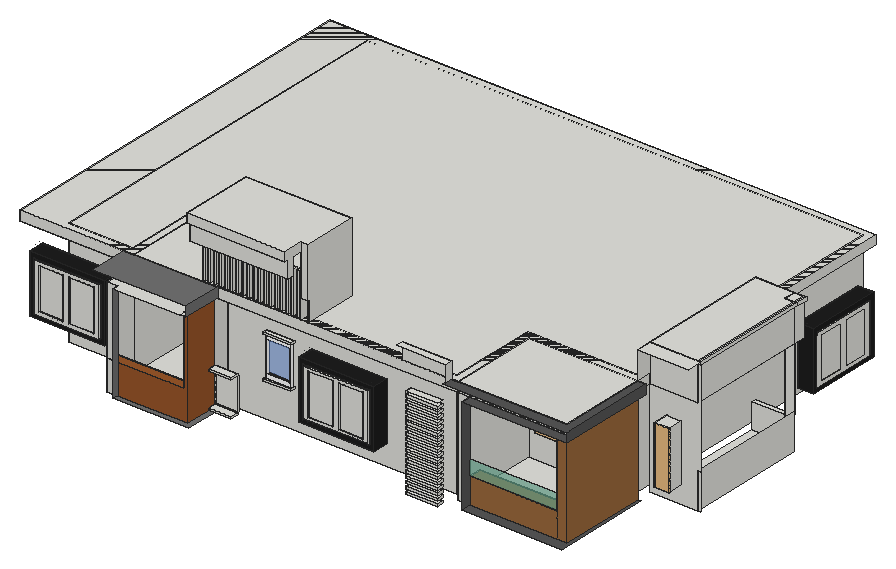
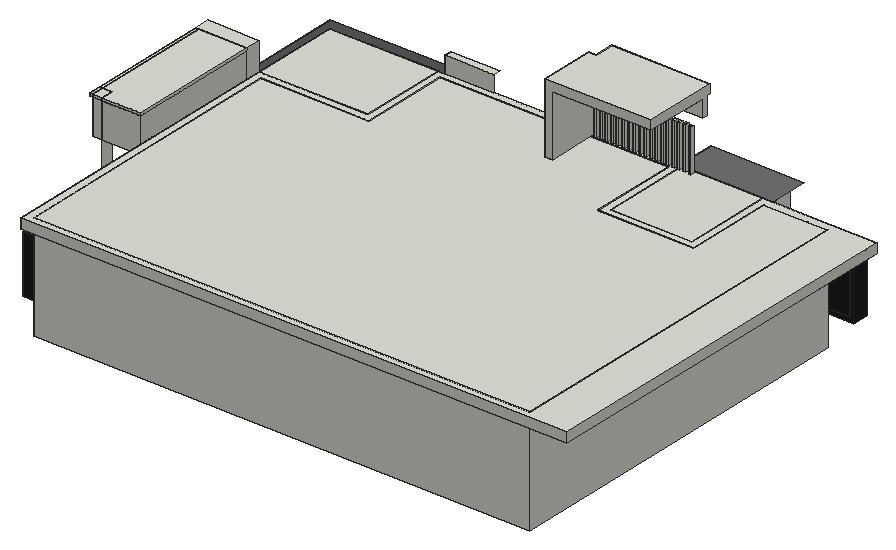
# SketchUp Ruby script. Lengths in inches.
U = 1.inch
M = Sketchup.active_model
def pt(a) = Geom::Point3d.new(a.map { |v| v * U })
def face(e, loops, mat)
  f = e.add_face(loops[0].map { |a| pt(a) })
  loops[1..].each { |l| e.add_face(l.map { |a| pt(a) }).erase! }
  f.material = f.back_material = mat if mat
  f
end
# faces: each face lists its corners as indices into pts; further lists are holes
def faces(e, pts, list, mat = nil) = list.each { |f| face(e, (f[0].is_a?(Array) ? f : [f]).map { |l| l.map { |i| pts[i] } }, mat) }
# xy, xz, yz: faces in a plane at the given z, y or x. An outline is a flat list of corners, or four numbers for a rectangle; further outlines are holes
def ring(l) = l.size == 4 ? [[l[0], l[1]], [l[2], l[1]], [l[2], l[3]], [l[0], l[3]]] : l.each_slice(2).to_a
def flat(e, list, mat, &to3) = list.each { |f| face(e, (f[0].is_a?(Array) ? f : [f]).map { |l| ring(l).map { |u, v| to3.(u, v) } }, mat) }
def xy(e, z, list, mat = nil) = flat(e, list, mat) { |x, y| [x, y, z] }
def xz(e, y, list, mat = nil) = flat(e, list, mat) { |x, z| [x, y, z] }
def yz(e, x, list, mat = nil) = flat(e, list, mat) { |y, z| [x, y, z] }
def lines(e, pts, list) = list.each { |a, b| e.add_line(pt(pts[a]), pt(pts[b])) }
# prism: a flat outline (further loops are holes) pulled along v
def prism(e, loops, v, mat = nil)
  f = face(e, loops, mat); d = Geom::Vector3d.new(v.map { |x| x * U })
  f.pushpull(f.normal.samedirection?(d) ? d.length : -d.length)
end
def box(e, o, s, mat = nil) = prism(e, [[o, [o[0] + s[0], o[1], o[2]], [o[0] + s[0], o[1] + s[1], o[2]], [o[0], o[1] + s[1], o[2]]]], [0, 0, s[2]], mat)
def at(x, y, z, deg = 0) = Geom::Transformation.translation(pt([x, y, z])) * Geom::Transformation.rotation(ORIGIN, Z_AXIS, deg.degrees)
def axes(o, x, y, z) = Geom::Transformation.new([*x, 0, *y, 0, *z, 0, *pt(o).to_a, 1])
def part(name) = M.definitions.add(name)
# library, detail: a bought-in or finely detailed component or shape, given as its bounding box
def library(name, o, s) = part(name).tap { |d| box(d.entities, o, s) }
def detail(e, o, s) = box(e.add_group.entities, o, s)
def put(e, d, t, mat = nil) = e.add_instance(d, t).tap { |i| i.material = mat if mat }
def group(e, t, mat = nil) = e.add_group.tap { |g| g.transformation = t; g.material = mat if mat }.entities
root = M.entities
M.materials.add("MaterialE").color = [182, 131, 172]
M.materials["MaterialE"].alpha = 0.66
M.materials.add("MaterialF").color = [114, 188, 161]
M.materials["MaterialF"].alpha = 0.66
M.materials.add("[Color M05]").color = [114, 114, 114]
M.materials.add("[Color M06]").color = [86, 86, 86]
M.materials.add("[Color M08]").color = [30, 30, 30]
M.materials.add("[Color_000]").color = [255, 255, 255]
M.materials.add("[Translucent Glass Blue]").color = [100, 149, 237]
M.materials["[Translucent Glass Blue]"].alpha = 0.5
M.materials.add("[Wood Cherry Original]").color = [152, 86, 42]
M.materials.add("[Wood Floor]").color = [155, 105, 61]
c1 = part("Group\#4")
box(c1.entities,[0,0,0],[39.5625,8.625,2.78])
c2 = part("Group\#75")
box(c2.entities,[0,-10.375,0],[28.375,10.375,2.5])
c3 = library("Single door",[0,0,0],[7.5,39.86,83.92])
c4 = part("Window")
xy(c4.entities,31.72,[[-0.78,88.6,2.72,128.1]])
xy(c4.entities,34.95,[[-0.78,91.53,0.84,106.59],[0.84,91.53,1.05,97.58],[1.05,91.53,1.42,106.59],[1.42,91.53,2.72,106.59],[0.84,97.58,1.05,98.18],
  [0.84,98.18,1.05,106.59]])
xy(c4.entities,35.27,[[-0.78,110.09,0.97,125.14],[1.05,110.09,2.72,125.14]])
xy(c4.entities,58.35,[[2.72,108.74,3.8,109.74]])
xy(c4.entities,77.8125,[[-0.78,110.09,2.72,125.14],[0.97,110.09,1.05,125.14]])
xy(c4.entities,77.93,[[-0.78,91.53,0.84,106.59],[1.05,91.53,1.42,106.59],[1.42,91.53,2.72,106.59]])
xy(c4.entities,80.72,[[-0.78,88.6,2.72,128.1]])
xz(c4.entities,88.6,[[-0.78,31.72,2.72,80.72]])
xz(c4.entities,91.53,[[-0.78,34.95,0.84,77.93],[1.05,34.95,1.42,77.93],[1.42,34.95,2.72,77.93]])
xz(c4.entities,106.59,[[-0.78,34.95,0.84,77.93],[0.84,34.95,1.05,77.93],[0.84,34.95,2.72,77.93]])
xz(c4.entities,108.74,[[3.8,54.35,4.22,54.6,4.22,59.47,2.72,59.97,2.72,58.35,3.8,58.35]])
xz(c4.entities,109.74,[[3.8,54.35,3.8,58.35,2.72,58.35,2.72,59.97,4.22,59.47,4.22,54.6]])
xz(c4.entities,110.09,[[-0.78,35.27,0.97,77.8125],[1.05,35.27,2.72,77.8125]])
xz(c4.entities,125.14,[[-0.78,35.27,0.97,77.8125],[0.97,35.27,1.05,80.72],[1.05,35.27,2.72,77.8125]])
xz(c4.entities,128.1,[[-0.78,31.72,2.72,80.72]])
yz(c4.entities,-0.78,[[[88.6,31.72,128.1,80.72],[91.53,34.95,106.59,77.93],[110.09,35.27,125.14,77.8125]]])
yz(c4.entities,0.84,[[91.53,34.95,106.59,77.93]])
yz(c4.entities,0.97,[[110.09,35.27,125.14,77.8125]])
yz(c4.entities,1.05,[[91.53,34.95,106.59,77.93],[110.09,35.27,125.14,77.8125]])
yz(c4.entities,1.42,[[91.53,34.95,106.59,77.93]])
yz(c4.entities,2.72,[[[88.6,31.72,108.35,80.72],[91.53,34.95,106.59,77.93]],[[108.35,31.72,128.1,80.72],[110.09,35.27,125.14,77.8125],[108.74,58.35,109.74,59.97]]])
yz(c4.entities,3.8,[[108.74,54.35,109.74,58.35]])
yz(c4.entities,4.22,[[108.74,54.6,109.74,59.47]])
p = [[4.22,108.74,54.6],[3.8,108.74,54.35],[3.8,109.74,54.35],[4.22,109.74,54.6],[2.72,109.74,59.97],[2.72,108.74,59.97],
  [4.22,108.74,59.47],[4.22,109.74,59.47],[-0.78,86.4,89.94],[-0.78,86.44,89.94],[15.22,130.69,89.94],[15.22,130.65,89.94],
  [-0.78,86.44,28.19],[-0.78,86.4,28.19],[7.72,130.69,89.94],[7.72,130.65,89.94]]
faces(c4.entities,p,[[0,1,2,3],[4,5,6,7]])
lines(c4.entities,p,[[8,9],[10,11],[12,13],[14,15]])
c5 = part("Group\#5")
xy(c5.entities,0,[[[0,0,93.5,72.0625],[5.4,5.4,88.1,66.66]],[5.4,5.4,88.1,66.66]])
xy(c5.entities,20.1875,[[[0,0,93.5,72.0625],[5.4,5.4,88.1,66.66]]])
xz(c5.entities,0,[[0,0,93.5,20.1875]])
xz(c5.entities,5.4,[[5.4,0,88.1,20.1875]])
xz(c5.entities,66.66,[[5.4,0,88.1,20.1875]])
xz(c5.entities,72.0625,[[0,0,93.5,20.1875]])
yz(c5.entities,0,[[0,0,72.0625,20.1875]])
yz(c5.entities,5.4,[[5.4,0,66.66,20.1875]])
yz(c5.entities,88.1,[[5.4,0,66.66,20.1875]])
yz(c5.entities,93.5,[[0,0,72.0625,20.1875]])
c6 = library("grille P1",[0,0,0],[0.79,28.9,72.83])
c7 = part("glassE")
xy(c7.entities,0,[[0,0,37.99,0.79]],"MaterialE")
xy(c7.entities,38.27,[[0,0,37.99,0.79]],"MaterialE")
xz(c7.entities,0,[[0,0,37.99,38.27]],"MaterialF")
yz(c7.entities,0,[[0,0,0.79,38.27]],"MaterialE")
yz(c7.entities,37.99,[[0,0,0.79,38.27]],"MaterialE")
c8 = library("Sliding Window",[0,0,0],[35.43,4.93,59.06])
c9 = part("Group\#73")
box(c9.entities,[0,0,0],[34.1875,2.25,6.125])
c10 = part("bod vindu")
g1 = group(c10.entities,at(0,-46.85,0),"[Translucent Glass Blue]")
yz(g1,0.94,[[2.36,2.36,44.49,19.65]],"[Translucent Glass Blue]")
p = [[0.55,44.49,2.36],[0.94,44.49,2.36],[0.55,2.36,19.65],[0.94,2.36,19.65]]
lines(g1,p,[[0,1],[2,3]])
g2 = group(g1,at(0,46.85,0,-90),"[Color_000]")
xy(g2,0,[[0,0,46.85,3.9375]])
xy(g2,1.57,[[1.57,0,45.28,0.55]])
xy(g2,2.36,[[2.36,0.55,44.49,3.9375]])
xy(g2,19.65,[[2.36,0.55,4.29,3.9375],[4.29,0.55,44.49,3.9375]])
xy(g2,20.43,[[1.57,0,45.28,0.55]])
xy(g2,22.01,[[0,0,46.85,3.9375]])
xz(g2,0,[[[0,0,46.85,22.01],[1.57,1.57,45.28,20.43]]])
xz(g2,0.55,[[1.57,1.57,45.28,2.36],[1.57,2.36,2.36,2.36,2.36,19.65,44.49,19.65,44.49,2.36,45.28,2.36,45.28,20.43,1.57,20.43]])
xz(g2,3.9375,[[[0,0,46.85,22.01],[2.36,2.36,44.49,19.65]]])
yz(g2,0,[[0,0,3.9375,22.01]])
yz(g2,1.57,[[0,1.57,0.55,2.36,0.55,20.43,0,20.43]])
yz(g2,2.36,[[0.55,2.36,3.9375,19.65]])
yz(g2,44.49,[[0.55,2.36,3.9375,19.65]])
yz(g2,45.28,[[0,1.57,0,20.43,0.55,20.43,0.55,2.36]])
yz(g2,46.85,[[0,0,3.9375,22.01]])
p = [[45.28,0,1.57],[1.57,0,1.57],[1.57,0.55,2.36],[2.36,0.55,2.36],[44.49,0.55,2.36],[45.28,0.55,2.36]]
faces(g2,p,[[0,1,2,3,4,5]])
xy(root,394.01,[[304.51,155.5,398.77,155.5,398.77,203.9375,392.02,203.9375,392.02,162.1875,291.51,162.1875,291.51,162.06,304.51,162.06]],"[Color M05]")
xy(root,396,[[291.51,172.6875,386.62,172.6875,386.62,203.9375,392.02,203.9375,392.02,313.75,291.32,313.75,291.32,203.9375,291.51,203.9375],[693.39,203.9375,707.82,203.9375,707.82,219.8125,816.38,219.8125,816.38,313.75,693.39,313.75],[203.47,212.9375,282.32,212.9375,282.32,322.75,401.02,322.75,401.02,212.9375,684.39,212.9375,684.39,322.75,818.97,322.75,818.97,674.9375,203.47,674.9375],[827.97,332.62,882.11,332.62,882.11,481.58,876.25,481.58,876.25,490.94,827.97,490.94],[882.11,332.62,887.97,481.58]])
xy(root,396,[[707.95,190.6875,832.47,190.6875,832.47,313.75,827.97,313.75,827.97,203.9375,707.95,203.9375]],"[Color M06]")
xy(root,397.79,[[392.02,203.9375,420.4,205.4375]])
xy(root,417.54,[[848.78,313.75,867.09,332.62]])
xy(root,426.875,[[827.97,490.94,876.25,496.51]])
xy(root,428,[[707.82,203.9375,816.38,219.8125]],"[Wood Floor]")
xy(root,432,[[291.51,162.1875,386.62,172.6875]],"[Wood Cherry Original]")
xy(root,438.17,[[392.02,203.9375,420.4,205.4375]])
xy(root,488.67,[[848.78,313.75,867.09,332.62]])
xy(root,501.53,[[635.73,194.4375,675.23,203.0625]])
xy(root,516,[[304.51,155.5,304.51,162.06,291.51,162.06,291.51,203.9375,386.62,203.9375,386.62,155.5],[386.62,155.5,392.02,162.1875],[386.62,162.1875,392.02,183],[386.62,183,392.02,203.9375],[816.38,203.9375,827.97,313.75],
  [827.97,332.62,887.97,496.51]])
xy(root,516,[[392.02,155.5,395.02,203.9375]],"[Color M05]")
xy(root,516,[[707.95,190.6875,707.95,203.9375,827.97,203.9375,827.97,313.75,838.2,313.75,838.2,190.6875]],"[Color M06]")
xy(root,528,[[[150.47,203.9375,291.32,203.9375,291.32,313.75,392.02,313.75,392.02,203.9375,693.39,203.9375,693.39,313.75,827.97,313.75,827.97,683.9375,150.47,683.9375],[203.47,212.9375,203.47,674.9375,818.97,674.9375,818.97,322.75,684.39,322.75,684.39,212.9375,401.02,212.9375,401.02,322.75,282.32,322.75,282.32,212.9375]],[497.83,203.9375,507.4,212.9375],[497.83,212.9375,507.4,271.6875]])
xy(root,528,[[278.57,155.5,395.02,203.9375]],"[Color M05]")
xy(root,528,[[685.61,190.6875,838.2,190.6875,838.2,313.75,827.97,313.75,827.97,203.9375,685.61,203.9375]],"[Color M06]")
xy(root,548.1875,[[624.38,194.4375,685.61,203.9375]])
xy(root,559.3125,[[827.97,332.62,827.97,496.51,876.25,496.51,876.25,481.58,887.97,481.58,887.97,332.62],[887.97,332.62,891.78,481.58],[876.25,481.58,887.97,496.51],[887.97,481.58,891.78,496.51]])
xy(root,562.75,[[827.97,313.75,891.78,332.62],[827.97,332.62,887.97,332.62,887.97,481.58,876.25,481.58,876.25,496.51,827.97,496.51],[887.97,332.62,891.78,481.58],[876.25,481.58,887.97,496.51],[887.97,481.58,891.78,496.51]])
xy(root,581.5,[[375.96,184.61,497.83,191.78]])
xy(root,603.3125,[[375.96,179.625,497.83,184.61],[375.96,191.78,497.83,203.9375],[375.96,203.9375,497.83,271.6875]])
xy(root,614.4375,[[375.96,179.625,497.83,179.625,497.83,203.9375,507.4,203.9375,507.4,271.6875,375.96,271.6875]])
xz(root,162.06,[[291.51,394.01,304.51,432],[291.51,432,304.51,516]])
xz(root,162.1875,[[291.51,394.01,392.02,394.01,392.02,516,386.62,516,386.62,432,291.51,432]],"[Wood Cherry Original]")
xz(root,172.6875,[[291.51,396,386.62,432]])
xz(root,179.625,[[375.96,603.3125,497.83,614.4375]])
xz(root,184.61,[[375.96,581.5,497.83,603.3125]])
xz(root,191.78,[[375.96,581.5,497.83,603.3125]])
xz(root,203.9375,[[291.32,396,291.32,528,392.02,528,392.02,516,291.51,516,291.51,396],[386.62,396,392.02,516],[693.39,396,693.39,528,827.97,528,827.97,516,707.95,516,707.95,428,707.82,428,707.82,396],[392.02,516,395.02,528],[507.4,528,508.2,552.375],
  [624.38,528,685.61,548.1875],[497.83,552.375,507.4,614.4375]])
xz(root,203.9375,[[707.95,396,816.38,428],[816.38,396,827.97,516]],"[Wood Floor]")
xz(root,205.4375,[[392.02,397.79,420.4,438.17]])
xz(root,212.9375,[[203.47,396,282.32,528],[401.02,396,684.39,528]])
xz(root,219.8125,[[707.82,396,816.38,428]])
xz(root,271.6875,[[497.83,528,497.83,603.3125,375.96,603.3125,375.96,614.4375,507.4,614.4375,507.4,528]])
xz(root,313.75,[[291.32,396,392.02,528],[693.39,396,816.38,528],[816.38,516,827.97,528]])
xz(root,313.75,[[827.97,516,838.2,528]],"[Color M06]")
xz(root,322.75,[[282.32,396,401.02,528],[684.39,396,818.97,528]])
xz(root,332.62,[[[827.97,396,827.97,516,887.97,516,887.97,559.3125,891.78,559.3125,891.78,441.07,887.97,441.07,887.97,396],[848.78,417.54,867.09,488.67]],[887.97,396,891.78,441.07],[827.97,516,887.97,559.3125],[827.97,559.3125,887.97,562.75],[887.97,559.3125,891.78,562.75]])
xz(root,481.58,[[876.25,396,887.97,559.3125],[876.25,559.3125,887.97,562.75],[887.97,559.3125,891.78,562.75]])
xz(root,490.94,[[827.97,396,876.25,426.875]])
xz(root,496.51,[[827.97,516,876.25,559.3125],[876.25,516,887.97,559.3125],[827.97,559.3125,876.25,562.75],[876.25,559.3125,887.97,562.75],[887.97,559.3125,891.78,562.75]])
xz(root,674.9375,[[203.47,396,818.97,528]])
yz(root,203.47,[[212.9375,396,674.9375,528]])
yz(root,282.32,[[212.9375,396,322.75,528]])
yz(root,291.32,[[203.9375,396,313.75,528]])
yz(root,291.51,[[162.06,394.01,162.1875,432],[172.6875,396,203.9375,396,203.9375,516,162.06,516,162.06,432,172.6875,432]])
yz(root,304.51,[[155.5,394.01,162.06,516]],"[Color M05]")
yz(root,375.96,[[184.61,581.5,184.61,603.3125,179.625,603.3125,179.625,614.4375,271.6875,614.4375,271.6875,603.3125,191.78,603.3125,191.78,581.5]])
yz(root,386.62,[[172.6875,396,172.6875,432,162.1875,432,162.1875,516,203.9375,516,203.9375,396]])
yz(root,392.02,[[203.9375,396,203.9375,397.79,205.4375,397.79,205.4375,438.17,203.9375,438.17,203.9375,528,313.75,528,313.75,396],[203.9375,397.79,205.4375,438.17],[203.9375,397.79,205.4375,438.17]])
yz(root,392.02,[[162.1875,394.01,203.9375,516]],"[Wood Cherry Original]")
yz(root,395.02,[[155.5,516,203.9375,528]],"[Color M05]")
yz(root,401.02,[[212.9375,396,322.75,528]])
yz(root,420.4,[[203.9375,397.79,205.4375,438.17]])
yz(root,497.83,[[203.9375,528,271.6875,603.3125],[184.61,581.5,191.78,581.5,191.78,603.3125,203.9375,603.3125,203.9375,614.4375,179.625,614.4375,179.625,603.3125,184.61,603.3125]])
yz(root,507.4,[[203.9375,528,271.6875,614.4375]])
yz(root,635.73,[[194.4375,497.67,203.0625,501.53]])
yz(root,684.39,[[212.9375,396,322.75,528]])
yz(root,685.61,[[194.4375,528,203.9375,548.1875]])
yz(root,693.39,[[203.9375,396,313.75,528]])
yz(root,707.82,[[203.9375,396,219.8125,428]])
yz(root,707.95,[[190.6875,396,203.9375,516]],"[Color M06]")
yz(root,816.38,[[219.8125,396,219.8125,428,203.9375,428,203.9375,516,313.75,516,313.75,396]],"[Wood Floor]")
yz(root,818.97,[[322.75,396,674.9375,528]])
yz(root,827.97,[[203.9375,516,313.75,528],[332.62,516,496.51,528],[313.75,528,332.62,562.75],[332.62,528,496.51,559.3125],[332.62,559.3125,496.51,562.75]])
yz(root,827.97,[[203.9375,396,313.75,516]],"[Wood Floor]")
yz(root,838.2,[[190.6875,516,313.75,528]],"[Color M06]")
yz(root,848.78,[[313.75,417.54,332.62,488.67]])
yz(root,867.09,[[313.75,417.54,332.62,488.67]])
yz(root,876.25,[[481.58,396,481.58,559.3125,496.51,559.3125,496.51,426.875,490.94,426.875,490.94,396],[481.58,559.3125,496.51,562.75]])
yz(root,887.97,[[332.62,396,481.58,441.07],[332.62,516,481.58,559.3125],[481.58,516,496.51,559.3125],[332.62,559.3125,481.58,562.75],[481.58,559.3125,496.51,562.75]])
yz(root,891.78,[[332.62,559.3125,481.58,562.75],[481.58,559.3125,496.51,562.75]])
p = [[291.32,203.9375,516],[291.51,183,516]]
lines(root,p,[[0,1]])
put(root,c1,at(635.73,194.4375,386.88))
put(root,c1,at(635.73,194.4375,392.88))
put(root,c2,at(392.02,203.9375,395.29))
put(root,c1,at(635.73,194.4375,398.88))
put(root,c3,at(760.44,316.08,402,-90))
put(root,c1,at(635.73,194.4375,404.88))
put(root,c1,at(635.73,194.4375,410.88))
put(root,c4,axes([852.91,821.1,381.7],[-1,0,0],[0,-2.03871,0],[0,0,1.22883]))
put(root,c5,axes([833.5,554.66,416.34],[0,1,0],[0,0,1],[1,0,0]),"[Color M08]")
put(root,c1,at(635.73,194.4375,416.88))
put(root,c6,axes([867.09,313.75,417.29],[0,1,0],[-0.61577,0,0],[0,0,0.98]))
put(root,c1,at(635.73,194.4375,422.88))
put(root,c7,axes([707.95,203.9375,428],[2.85399,0,0],[0,1.17,0],[0,0,0.5016]))
put(root,c4,axes([778.5,184.53,393.73],[0,1,0],[-2.03871,0,0],[0,0,1.22883]))
put(root,c4,axes([444.25,184.53,393.73],[0,1,0],[-2.03871,0,0],[0,0,1.22883]))
put(root,c5,axes([512.06,203.9375,428.37],[1,0,0],[0,0,1],[0,-1,0]),"[Color M08]")
put(root,c5,axes([177.81,203.9375,428.37],[1,0,0],[0,0,1],[0,-1,0]),"[Color M08]")
put(root,c1,at(635.73,194.4375,428.88))
put(root,c8,at(704.35,308.67,429.25))
put(root,c1,at(635.73,194.4375,434.88))
put(root,c2,at(392.02,203.9375,438.17))
put(root,c1,at(635.73,194.4375,440.88))
put(root,c1,at(635.73,194.4375,446.88))
put(root,c9,axes([456.17,203.9375,448.49],[1,0,0],[0,0,1],[0,-1,0]))
put(root,c10,axes([488.85,203.9375,450.74],[0,-1,0],[0.6656,0,0],[0,0,2.2308]))
put(root,c1,at(635.73,194.4375,452.88))
put(root,c1,at(635.73,194.4375,458.88))
put(root,c1,at(635.73,194.4375,464.88))
put(root,c1,at(635.73,194.4375,470.88))
put(root,c1,at(635.73,194.4375,476.88))
put(root,c1,at(635.73,194.4375,482.88))
put(root,c1,at(635.73,194.4375,488.88))
put(root,c1,at(635.73,194.4375,494.88))
put(root,c9,axes([456.17,203.9375,499.83],[1,0,0],[0,0,1],[0,-1,0]))
g3 = group(root,at(193.09,683.9375,516))
xy(g3,0,[[-42.625,-480,634.875,0]])
xy(g3,12,[[[-42.625,-480,634.875,0],[298.35,-477.7,301.85,-473.08],[291.47,-477.7,294.97,-473.08],[284.6,-477.7,288.1,-473.08],[277.72,-477.7,281.22,-473.08],[270.85,-477.7,274.35,-473.08],[263.97,-477.7,267.47,-473.08],[257.1,-477.7,260.6,-473.08],[250.22,-477.7,253.72,-473.08],[243.35,-477.7,246.85,-473.08],[236.47,-477.7,239.97,-473.08],[229.6,-477.7,233.1,-473.08],[222.72,-477.7,226.22,-473.08],[215.85,-477.7,219.35,-473.08],[208.97,-477.7,212.47,-473.08],[202.1,-477.7,205.6,-473.08],[195.22,-477.7,198.72,-473.08],[188.35,-477.7,191.85,-473.08],[181.47,-477.7,184.97,-473.08]]])
xy(g3,64.375,[[181.47,-477.7,184.97,-473.08],[188.35,-477.7,191.85,-473.08],[195.22,-477.7,198.72,-473.08],[202.1,-477.7,205.6,-473.08],[208.97,-477.7,212.47,-473.08],
  [215.85,-477.7,219.35,-473.08],[222.72,-477.7,226.22,-473.08],[229.6,-477.7,233.1,-473.08],[236.47,-477.7,239.97,-473.08],[243.35,-477.7,246.85,-473.08],
  [250.22,-477.7,253.72,-473.08],[257.1,-477.7,260.6,-473.08],[263.97,-477.7,267.47,-473.08],[270.85,-477.7,274.35,-473.08],[277.72,-477.7,281.22,-473.08],
  [284.6,-477.7,288.1,-473.08],[291.47,-477.7,294.97,-473.08],[298.35,-477.7,301.85,-473.08]])
xz(g3,-480,[[-42.625,0,634.875,12]])
xz(g3,-477.7,[[181.47,12,184.97,64.375],[188.35,12,191.85,64.375],[195.22,12,198.72,64.375],[202.1,12,205.6,64.375],[208.97,12,212.47,64.375],
  [215.85,12,219.35,64.375],[222.72,12,226.22,64.375],[229.6,12,233.1,64.375],[236.47,12,239.97,64.375],[243.35,12,246.85,64.375],
  [250.22,12,253.72,64.375],[257.1,12,260.6,64.375],[263.97,12,267.47,64.375],[270.85,12,274.35,64.375],[277.72,12,281.22,64.375],
  [284.6,12,288.1,64.375],[291.47,12,294.97,64.375],[298.35,12,301.85,64.375]])
xz(g3,-473.08,[[181.47,12,184.97,64.375],[188.35,12,191.85,64.375],[195.22,12,198.72,64.375],[202.1,12,205.6,64.375],[208.97,12,212.47,64.375],
  [215.85,12,219.35,64.375],[222.72,12,226.22,64.375],[229.6,12,233.1,64.375],[236.47,12,239.97,64.375],[243.35,12,246.85,64.375],
  [250.22,12,253.72,64.375],[257.1,12,260.6,64.375],[263.97,12,267.47,64.375],[270.85,12,274.35,64.375],[277.72,12,281.22,64.375],
  [284.6,12,288.1,64.375],[291.47,12,294.97,64.375],[298.35,12,301.85,64.375]])
xz(g3,0,[[-42.625,0,634.875,12]])
yz(g3,-42.625,[[-480,0,0,12]])
yz(g3,181.47,[[-477.7,12,-473.08,64.375]])
yz(g3,184.97,[[-477.7,12,-473.08,64.375]])
yz(g3,188.35,[[-477.7,12,-473.08,64.375]])
yz(g3,191.85,[[-477.7,12,-473.08,64.375]])
yz(g3,195.22,[[-477.7,12,-473.08,64.375]])
yz(g3,198.72,[[-477.7,12,-473.08,64.375]])
yz(g3,202.1,[[-477.7,12,-473.08,64.375]])
yz(g3,205.6,[[-477.7,12,-473.08,64.375]])
yz(g3,208.97,[[-477.7,12,-473.08,64.375]])
yz(g3,212.47,[[-477.7,12,-473.08,64.375]])
yz(g3,215.85,[[-477.7,12,-473.08,64.375]])
yz(g3,219.35,[[-477.7,12,-473.08,64.375]])
yz(g3,222.72,[[-477.7,12,-473.08,64.375]])
yz(g3,226.22,[[-477.7,12,-473.08,64.375]])
yz(g3,229.6,[[-477.7,12,-473.08,64.375]])
yz(g3,233.1,[[-477.7,12,-473.08,64.375]])
yz(g3,236.47,[[-477.7,12,-473.08,64.375]])
yz(g3,239.97,[[-477.7,12,-473.08,64.375]])
yz(g3,243.35,[[-477.7,12,-473.08,64.375]])
yz(g3,246.85,[[-477.7,12,-473.08,64.375]])
yz(g3,250.22,[[-477.7,12,-473.08,64.375]])
yz(g3,253.72,[[-477.7,12,-473.08,64.375]])
yz(g3,257.1,[[-477.7,12,-473.08,64.375]])
yz(g3,260.6,[[-477.7,12,-473.08,64.375]])
yz(g3,263.97,[[-477.7,12,-473.08,64.375]])
yz(g3,267.47,[[-477.7,12,-473.08,64.375]])
yz(g3,270.85,[[-477.7,12,-473.08,64.375]])
yz(g3,274.35,[[-477.7,12,-473.08,64.375]])
yz(g3,277.72,[[-477.7,12,-473.08,64.375]])
yz(g3,281.22,[[-477.7,12,-473.08,64.375]])
yz(g3,284.6,[[-477.7,12,-473.08,64.375]])
yz(g3,288.1,[[-477.7,12,-473.08,64.375]])
yz(g3,291.47,[[-477.7,12,-473.08,64.375]])
yz(g3,294.97,[[-477.7,12,-473.08,64.375]])
yz(g3,298.35,[[-477.7,12,-473.08,64.375]])
yz(g3,301.85,[[-477.7,12,-473.08,64.375]])
yz(g3,634.875,[[-480,0,0,12]])
g4 = group(root,at(491.44,206.23,528))
xy(g4,0,[[0,0,3.5,4.625]])
g5 = group(root,at(494.82,185.58,581.5))
box(g5,[-3.875,0,0],[3.875,4.5625,1])
